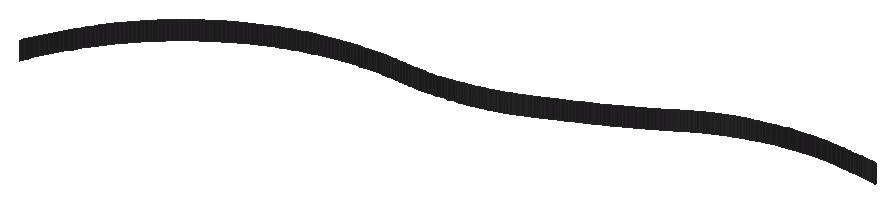
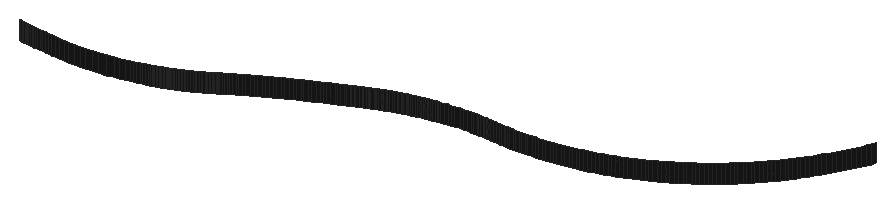
# SketchUp Ruby script. Lengths in inches.
U = 1.inch
M = Sketchup.active_model
def pt(a) = Geom::Point3d.new(a.map { |v| v * U })
def face(e, loops, mat)
  f = e.add_face(loops[0].map { |a| pt(a) })
  loops[1..].each { |l| e.add_face(l.map { |a| pt(a) }).erase! }
  f.material = f.back_material = mat if mat
  f
end
# faces: each face lists its corners as indices into pts; further lists are holes
def faces(e, pts, list, mat = nil) = list.each { |f| face(e, (f[0].is_a?(Array) ? f : [f]).map { |l| l.map { |i| pts[i] } }, mat) }
# xy, xz, yz: faces in a plane at the given z, y or x. An outline is a flat list of corners, or four numbers for a rectangle; further outlines are holes
def ring(l) = l.size == 4 ? [[l[0], l[1]], [l[2], l[1]], [l[2], l[3]], [l[0], l[3]]] : l.each_slice(2).to_a
def flat(e, list, mat, &to3) = list.each { |f| face(e, (f[0].is_a?(Array) ? f : [f]).map { |l| ring(l).map { |u, v| to3.(u, v) } }, mat) }
def xy(e, z, list, mat = nil) = flat(e, list, mat) { |x, y| [x, y, z] }
def xz(e, y, list, mat = nil) = flat(e, list, mat) { |x, z| [x, y, z] }
def yz(e, x, list, mat = nil) = flat(e, list, mat) { |y, z| [x, y, z] }
def lines(e, pts, list) = list.each { |a, b| e.add_line(pt(pts[a]), pt(pts[b])) }
# prism: a flat outline (further loops are holes) pulled along v
def prism(e, loops, v, mat = nil)
  f = face(e, loops, mat); d = Geom::Vector3d.new(v.map { |x| x * U })
  f.pushpull(f.normal.samedirection?(d) ? d.length : -d.length)
end
def box(e, o, s, mat = nil) = prism(e, [[o, [o[0] + s[0], o[1], o[2]], [o[0] + s[0], o[1] + s[1], o[2]], [o[0], o[1] + s[1], o[2]]]], [0, 0, s[2]], mat)
def at(x, y, z, deg = 0) = Geom::Transformation.translation(pt([x, y, z])) * Geom::Transformation.rotation(ORIGIN, Z_AXIS, deg.degrees)
def axes(o, x, y, z) = Geom::Transformation.new([*x, 0, *y, 0, *z, 0, *pt(o).to_a, 1])
def part(name) = M.definitions.add(name)
# library, detail: a bought-in or finely detailed component or shape, given as its bounding box
def library(name, o, s) = part(name).tap { |d| box(d.entities, o, s) }
def detail(e, o, s) = box(e.add_group.entities, o, s)
def put(e, d, t, mat = nil) = e.add_instance(d, t).tap { |i| i.material = mat if mat }
def group(e, t, mat = nil) = e.add_group.tap { |g| g.transformation = t; g.material = mat if mat }.entities
root = M.entities
M.materials.add("Marble_07_1K").color = [36, 34, 36]
xz(root,796.49,[[326.62,18,326.73,19],[326.73,18,326.84,19],[326.84,18,326.97,19]],"Marble_07_1K")
xz(root,796.5,[[326.25,18,326.34,19],[326.34,18,326.43,19],[326.43,18,326.52,19],[327.11,18,327.27,19]],"Marble_07_1K")
xz(root,796.51,[[326.07,18,326.16,19]],"Marble_07_1K")
xz(root,796.52,[[325.9,18,325.99,19]],"Marble_07_1K")
xz(root,796.53,[[325.73,18,325.82,19]],"Marble_07_1K")
xz(root,796.55,[[324.45,18,324.62,19],[325.4375,18,325.54,19]],"Marble_07_1K")
xz(root,796.56,[[324.78,18,324.93,19],[324.93,18,325.08,19],[325.08,18,325.21,19],[325.21,18,325.33,19]],"Marble_07_1K")
xz(root,802.3,[[347.43,18,347.47,19]],"Marble_07_1K")
xz(root,802.33,[[347.24,18,347.28,19]],"Marble_07_1K")
xz(root,802.34,[[347.16,18,347.2,19]],"Marble_07_1K")
xz(root,802.35,[[347.09,18,347.125,19]],"Marble_07_1K")
xz(root,802.36,[[347.01,18,347.05,19]],"Marble_07_1K")
xz(root,802.38,[[346.85,18,346.89,19]],"Marble_07_1K")
xz(root,802.39,[[346.74,18,346.8,19]],"Marble_07_1K")
xz(root,802.52,[[344.29,18,344.58,19]],"Marble_07_1K")
p = [[312.07,787.94,18],[311.99,787.75,18],[311.99,787.75,19],[312.07,787.94,19],[312.16,788.14,18],[312.16,788.14,19],
  [312.26,788.35,18],[312.26,788.35,19],[312.37,788.56,18],[312.37,788.56,19],[312.48,788.77,18],[312.48,788.77,19],
  [312.6,788.98,18],[312.6,788.98,19],[312.72,789.19,18],[312.72,789.19,19],[312.83,789.39,18],[312.83,789.39,19],
  [312.95,789.59,18],[312.95,789.59,19],[313.0625,789.78,18],[313.0625,789.78,19],[313.17,789.96,18],[313.17,789.96,19],
  [313.28,790.13,18],[313.28,790.13,19],[313.39,790.29,18],[313.39,790.29,19],[313.49,790.45,18],[313.49,790.45,19],
  [313.6,790.6,18],[313.6,790.6,19],[313.7,790.75,18],[313.7,790.75,19],[313.8125,790.9,18],[313.8125,790.9,19],
  [313.92,791.05,18],[313.92,791.05,19],[314.03,791.19,18],[314.03,791.19,19],[314.15,791.34,18],[314.15,791.34,19],
  [314.26,791.48,18],[314.26,791.48,19],[314.38,791.62,18],[314.38,791.62,19],[314.5,791.76,18],[314.5,791.76,19],
  [314.62,791.9,18],[314.62,791.9,19],[314.74,792.04,18],[314.74,792.04,19],[314.87,792.17,18],[314.87,792.17,19],
  [314.99,792.3,18],[314.99,792.3,19],[315.12,792.43,18],[315.12,792.43,19],[315.25,792.5625,18],[315.25,792.5625,19],
  [315.38,792.69,18],[315.38,792.69,19],[315.51,792.82,18],[315.51,792.82,19],[315.65,792.94,18],[315.65,792.94,19],
  [315.79,793.0625,18],[315.79,793.0625,19],[315.92,793.19,18],[315.92,793.19,19],[316.0625,793.3,18],[316.0625,793.3,19],
  [316.2,793.42,18],[316.2,793.42,19],[316.35,793.54,18],[316.35,793.54,19],[316.49,793.65,18],[316.49,793.65,19],
  [316.64,793.76,18],[316.64,793.76,19],[316.78,793.87,18],[316.78,793.87,19],[316.93,793.98,18],[316.93,793.98,19],
  [317.08,794.08,18],[317.08,794.08,19],[317.23,794.1875,18],[317.23,794.1875,19],[317.39,794.29,18],[317.39,794.29,19],
  [317.54,794.39,18],[317.54,794.39,19],[317.7,794.48,18],[317.7,794.48,19],[317.85,794.58,18],[317.85,794.58,19],
  [318.01,794.67,18],[318.01,794.67,19],[318.17,794.76,18],[318.17,794.76,19],[318.33,794.85,18],[318.33,794.85,19],
  [318.49,794.94,18],[318.49,794.94,19],[318.65,795.03,18],[318.65,795.03,19],[318.82,795.11,18],[318.82,795.11,19],
  [318.98,795.1875,18],[318.98,795.1875,19],[319.15,795.27,18],[319.15,795.27,19],[319.32,795.34,18],[319.32,795.34,19],
  [319.48,795.42,18],[319.48,795.42,19],[319.65,795.49,18],[319.65,795.49,19],[319.82,795.56,18],[319.82,795.56,19],
  [319.99,795.625,18],[319.99,795.625,19],[320.16,795.69,18],[320.16,795.69,19],[320.34,795.75,18],[320.34,795.75,19],
  [320.51,795.8125,18],[320.51,795.8125,19],[320.68,795.87,18],[320.68,795.87,19],[320.86,795.93,18],[320.86,795.93,19],
  [321.03,795.98,18],[321.03,795.98,19],[321.21,796.03,18],[321.21,796.03,19],[321.39,796.08,18],[321.39,796.08,19],
  [321.5625,796.125,18],[321.5625,796.125,19],[321.74,796.17,18],[321.74,796.17,19],[321.92,796.21,18],[321.92,796.21,19],
  [322.1,796.25,18],[322.1,796.25,19],[322.28,796.29,18],[322.28,796.29,19],[322.46,796.32,18],[322.46,796.32,19],
  [322.64,796.36,18],[322.64,796.36,19],[322.82,796.39,18],[322.82,796.39,19],[323,796.41,18],[323,796.41,19],
  [323.18,796.4375,18],[323.18,796.4375,19],[323.37,796.46,18],[323.37,796.46,19],[323.55,796.48,18],[323.55,796.48,19],
  [323.73,796.5,18],[323.73,796.5,19],[323.92,796.51,18],[323.92,796.51,19],[324.1,796.53,18],[324.1,796.53,19],
  [324.28,796.54,18],[324.28,796.54,19],[324.45,796.55,18],[324.45,796.55,19],[325.64,796.54,18],[325.54,796.55,18],
  [325.54,796.55,19],[325.64,796.54,19],[325.73,796.53,18],[325.73,796.53,19],[325.9,796.52,18],[325.82,796.53,18],
  [325.82,796.53,19],[325.9,796.52,19],[326.07,796.51,18],[325.99,796.52,18],[325.99,796.52,19],[326.07,796.51,19],
  [326.25,796.5,18],[326.16,796.51,18],[326.16,796.51,19],[326.25,796.5,19],[326.62,796.49,18],[326.52,796.5,18],
  [326.52,796.5,19],[326.62,796.49,19],[327.11,796.5,18],[326.97,796.49,18],[326.97,796.49,19],[327.11,796.5,19],
  [327.45,796.51,18],[327.27,796.5,18],[327.27,796.5,19],[327.45,796.51,19],[327.65,796.52,18],[327.65,796.52,19],
  [327.88,796.53,18],[327.88,796.53,19],[328.11,796.56,18],[328.11,796.56,19],[324.78,796.56,18],[324.62,796.55,18],
  [324.62,796.55,19],[324.78,796.56,19],[325.4375,796.55,18],[325.33,796.56,18],[325.33,796.56,19],[325.4375,796.55,19],
  [328.3125,796.58,18],[328.3125,796.58,19],[328.49,796.6,18],[328.49,796.6,19],[328.65,796.625,18],[328.65,796.625,19],
  [328.79,796.65,18],[328.79,796.65,19],[328.91,796.67,18],[328.91,796.67,19],[329.02,796.68,18],[329.02,796.68,19],
  [329.13,796.7,18],[329.13,796.7,19],[329.23,796.72,18],[329.23,796.72,19],[329.32,796.74,18],[329.32,796.74,19],
  [329.41,796.76,18],[329.41,796.76,19],[329.5,796.77,18],[329.5,796.77,19],[329.58,796.79,18],[329.58,796.79,19],
  [329.66,796.81,18],[329.66,796.81,19],[329.82,796.85,18],[329.74,796.83,18],[329.74,796.83,19],[329.82,796.85,19],
  [329.9,796.87,18],[329.9,796.87,19],[329.98,796.89,18],[329.98,796.89,19],[330.0625,796.91,18],[330.0625,796.91,19],
  [330.22,796.95,18],[330.14,796.93,18],[330.14,796.93,19],[330.22,796.95,19],[330.3,796.97,18],[330.3,796.97,19],
  [330.38,796.99,18],[330.38,796.99,19],[330.46,797.01,18],[330.46,797.01,19],[330.62,797.06,18],[330.54,797.04,18],
  [330.54,797.04,19],[330.62,797.06,19],[330.69,797.08,18],[330.69,797.08,19],[330.77,797.11,18],[330.77,797.11,19],
  [330.85,797.13,18],[330.85,797.13,19],[330.93,797.16,18],[330.93,797.16,19],[331.01,797.1875,18],[331.01,797.1875,19],
  [331.08,797.21,18],[331.08,797.21,19],[331.16,797.24,18],[331.16,797.24,19],[331.24,797.27,18],[331.24,797.27,19],
  [331.32,797.29,18],[331.32,797.29,19],[331.39,797.32,18],[331.39,797.32,19],[331.47,797.35,18],[331.47,797.35,19],
  [331.62,797.41,18],[331.55,797.38,18],[331.55,797.38,19],[331.62,797.41,19],[331.7,797.44,18],[331.7,797.44,19],
  [331.78,797.47,18],[331.78,797.47,19],[331.85,797.5,18],[331.85,797.5,19],[332,797.57,18],[331.93,797.54,18],
  [331.93,797.54,19],[332,797.57,19],[332.08,797.6,18],[332.08,797.6,19],[332.15,797.63,18],[332.15,797.63,19],
  [332.23,797.67,18],[332.23,797.67,19],[332.31,797.7,18],[332.31,797.7,19],[332.38,797.74,18],[332.38,797.74,19],
  [332.46,797.77,18],[332.46,797.77,19],[332.625,797.85,18],[332.54,797.8125,18],[332.54,797.8125,19],[332.625,797.85,19],
  [332.71,797.9,18],[332.71,797.9,19],[332.81,797.94,18],[332.81,797.94,19],[332.91,797.99,18],[332.91,797.99,19],
  [333.02,798.04,18],[333.02,798.04,19],[333.14,798.1,18],[333.14,798.1,19],[333.27,798.16,18],[333.27,798.16,19],
  [333.41,798.22,18],[333.41,798.22,19],[333.55,798.29,18],[333.55,798.29,19],[333.7,798.36,18],[333.7,798.36,19],
  [333.85,798.43,18],[333.85,798.43,19],[334.01,798.5,18],[334.01,798.5,19],[334.16,798.57,18],[334.16,798.57,19],
  [334.31,798.65,18],[334.31,798.65,19],[334.47,798.72,18],[334.47,798.72,19],[334.62,798.8,18],[334.62,798.8,19],
  [334.77,798.87,18],[334.77,798.87,19],[334.92,798.95,18],[334.92,798.95,19],[335.08,799.02,18],[335.08,799.02,19],
  [335.23,799.1,18],[335.23,799.1,19],[335.375,799.18,18],[335.375,799.18,19],[335.53,799.26,18],[335.53,799.26,19],
  [335.68,799.34,18],[335.68,799.34,19],[335.83,799.42,18],[335.83,799.42,19],[335.97,799.5,18],[335.97,799.5,19],
  [336.12,799.58,18],[336.12,799.58,19],[336.27,799.66,18],[336.27,799.66,19],[336.42,799.75,18],[336.42,799.75,19],
  [336.57,799.83,18],[336.57,799.83,19],[336.71,799.91,18],[336.71,799.91,19],[336.86,800,18],[336.86,800,19],
  [337,800.08,18],[337,800.08,19],[337.13,800.16,18],[337.13,800.16,19],[337.26,800.23,18],[337.26,800.23,19],
  [337.375,800.3,18],[337.375,800.3,19],[337.48,800.37,18],[337.48,800.37,19],[337.57,800.42,18],[337.57,800.42,19],
  [337.65,800.47,18],[337.65,800.47,19],[337.78,800.54,18],[337.72,800.51,18],[337.72,800.51,19],[337.78,800.54,19],
  [337.82,800.57,18],[337.82,800.57,19],[337.86,800.6,18],[337.86,800.6,19],[337.95,800.66,18],[337.93,800.64,18],
  [337.93,800.64,19],[337.95,800.66,19],[337.89,800.62,18],[337.89,800.62,19],[338.07,800.73,18],[338.04,800.71,18],
  [338.04,800.71,19],[338.07,800.73,19],[338.01,800.7,18],[338.01,800.7,19],[337.98,800.68,18],[337.98,800.68,19],
  [338.11,800.75,18],[338.11,800.75,19],[338.17,800.8,18],[338.14,800.77,18],[338.14,800.77,19],[338.17,800.8,19],
  [338.25,800.84,18],[338.21,800.82,18],[338.21,800.82,19],[338.25,800.84,19],[338.29,800.87,18],[338.29,800.87,19],
  [338.39,800.92,18],[338.34,800.89,18],[338.34,800.89,19],[338.39,800.92,19],[338.45,800.96,18],[338.45,800.96,19],
  [338.59,801.04,18],[338.52,801,18],[338.52,801,19],[338.59,801.04,19],[338.68,801.09,18],[338.68,801.09,19],
  [338.77,801.13,18],[338.77,801.13,19],[338.85,801.17,18],[338.85,801.17,19],[338.92,801.21,18],[338.92,801.21,19],
  [338.98,801.24,18],[338.98,801.24,19],[339.03,801.27,18],[339.03,801.27,19],[339.08,801.29,18],[339.08,801.29,19],
  [339.17,801.33,18],[339.125,801.3125,18],[339.125,801.3125,19],[339.17,801.33,19],[339.21,801.35,18],[339.21,801.35,19],
  [339.28,801.39,18],[339.24,801.37,18],[339.24,801.37,19],[339.28,801.39,19],[339.38,801.43,18],[339.35,801.42,18],
  [339.35,801.42,19],[339.38,801.43,19],[339.3125,801.4,18],[339.3125,801.4,19],[339.44,801.46,18],[339.41,801.45,18],
  [339.41,801.45,19],[339.44,801.46,19],[339.48,801.48,18],[339.48,801.48,19],[339.57,801.52,18],[339.54,801.5,18],
  [339.54,801.5,19],[339.57,801.52,19],[339.51,801.49,18],[339.51,801.49,19],[339.67,801.56,18],[339.64,801.54,18],
  [339.64,801.54,19],[339.67,801.56,19],[339.61,801.53,18],[339.61,801.53,19],[339.77,801.6,18],[339.74,801.59,18],
  [339.74,801.59,19],[339.77,801.6,19],[339.71,801.57,18],[339.71,801.57,19],[339.87,801.64,18],[339.84,801.625,18],
  [339.84,801.625,19],[339.87,801.64,19],[339.8,801.61,18],[339.8,801.61,19],[339.9,801.65,18],[339.9,801.65,19],
  [339.97,801.68,18],[339.94,801.66,18],[339.94,801.66,19],[339.97,801.68,19],[340.07,801.71,18],[340.03,801.7,18],
  [340.03,801.7,19],[340.07,801.71,19],[340,801.69,18],[340,801.69,19],[340.17,801.75,18],[340.13,801.74,18],
  [340.13,801.74,19],[340.17,801.75,19],[340.1,801.73,18],[340.1,801.73,19],[340.27,801.79,18],[340.23,801.77,18],
  [340.23,801.77,19],[340.27,801.79,19],[340.2,801.76,18],[340.2,801.76,19],[340.37,801.82,18],[340.33,801.81,18],
  [340.33,801.81,19],[340.37,801.82,19],[340.3,801.8,18],[340.3,801.8,19],[340.47,801.86,18],[340.44,801.84,18],
  [340.44,801.84,19],[340.47,801.86,19],[340.4,801.83,18],[340.4,801.83,19],[340.57,801.89,18],[340.54,801.88,18],
  [340.54,801.88,19],[340.57,801.89,19],[340.5,801.87,18],[340.5,801.87,19],[340.66,801.92,18],[340.61,801.9,18],
  [340.61,801.9,19],[340.66,801.92,19],[340.79,801.95,18],[340.72,801.93,18],[340.72,801.93,19],[340.79,801.95,19],
  [340.87,801.97,18],[340.87,801.97,19],[340.96,802,18],[340.96,802,19],[341.07,802.03,18],[341.07,802.03,19],
  [341.21,802.07,18],[341.21,802.07,19],[341.36,802.11,18],[341.36,802.11,19],[341.55,802.15,18],[341.55,802.15,19],
  [341.76,802.2,18],[341.76,802.2,19],[342.01,802.26,18],[342.01,802.26,19],[342.3,802.32,18],[342.3,802.32,19],
  [342.63,802.39,18],[342.63,802.39,19],[347.16,802.34,18],[347.125,802.35,18],[347.125,802.35,19],[347.16,802.34,19],
  [347.24,802.33,18],[347.2,802.34,18],[347.2,802.34,19],[347.24,802.33,19],[347.35,802.3125,18],[347.32,802.32,18],
  [347.32,802.32,19],[347.35,802.3125,19],[347.28,802.33,18],[347.28,802.33,19],[347.43,802.3,18],[347.39,802.31,18],
  [347.39,802.31,19],[347.43,802.3,19],[342.99,802.4375,18],[342.99,802.4375,19],[343.34,802.47,18],[343.34,802.47,19],
  [346.1,802.45,18],[345.9375,802.46,18],[345.9375,802.46,19],[346.1,802.45,19],[346.25,802.4375,18],[346.25,802.4375,19],
  [346.38,802.43,18],[346.38,802.43,19],[346.49,802.42,18],[346.49,802.42,19],[346.59,802.41,18],[346.59,802.41,19],
  [346.67,802.4,18],[346.67,802.4,19],[346.74,802.39,18],[346.74,802.39,19],[346.85,802.38,18],[346.8,802.39,18],
  [346.8,802.39,19],[346.85,802.38,19],[346.97,802.37,18],[346.93,802.375,18],[346.93,802.375,19],[346.97,802.37,19],
  [346.89,802.38,18],[346.89,802.38,19],[347.09,802.35,18],[347.05,802.36,18],[347.05,802.36,19],[347.09,802.35,19],
  [347.01,802.36,18],[347.01,802.36,19],[343.67,802.5,18],[343.67,802.5,19],[343.99,802.51,18],[343.99,802.51,19],
  [344.29,802.52,18],[344.29,802.52,19],[344.85,802.51,18],[344.58,802.52,18],[344.58,802.52,19],[344.85,802.51,19],
  [345.11,802.5,18],[345.11,802.5,19],[345.34,802.49,18],[345.34,802.49,19],[345.56,802.48,18],[345.56,802.48,19],
  [345.76,802.47,18],[345.76,802.47,19]]
faces(root,p,[[0,1,2,3],[4,0,3,5],[6,4,5,7],[8,6,7,9],[10,8,9,11],[12,10,11,13],[14,12,13,15],[16,14,15,17],
  [18,16,17,19],[20,18,19,21],[22,20,21,23],[24,22,23,25],[26,24,25,27],[28,26,27,29],[30,28,29,31],[32,30,31,33],
  [34,32,33,35],[36,34,35,37],[38,36,37,39],[40,38,39,41],[42,40,41,43],[44,42,43,45],[46,44,45,47],[48,46,47,49],
  [50,48,49,51],[52,50,51,53],[54,52,53,55],[56,54,55,57],[58,56,57,59],[60,58,59,61],[62,60,61,63],[64,62,63,65],
  [66,64,65,67],[68,66,67,69],[70,68,69,71],[72,70,71,73],[74,72,73,75],[76,74,75,77],[78,76,77,79],[80,78,79,81],
  [82,80,81,83],[84,82,83,85],[86,84,85,87],[88,86,87,89],[90,88,89,91],[92,90,91,93],[94,92,93,95],[96,94,95,97],
  [98,96,97,99],[100,98,99,101],[102,100,101,103],[104,102,103,105],[106,104,105,107],[108,106,107,109],[110,108,109,111],[112,110,111,113],
  [114,112,113,115],[116,114,115,117],[118,116,117,119],[120,118,119,121],[122,120,121,123],[124,122,123,125],[126,124,125,127],[128,126,127,129],
  [130,128,129,131],[132,130,131,133],[134,132,133,135],[136,134,135,137],[138,136,137,139],[140,138,139,141],[142,140,141,143],[144,142,143,145],
  [146,144,145,147],[148,146,147,149],[150,148,149,151],[152,150,151,153],[154,152,153,155],[156,154,155,157],[158,156,157,159],[160,158,159,161],
  [162,160,161,163],[164,162,163,165],[166,164,165,167],[168,166,167,169],[170,168,169,171],[172,173,174,175],[176,172,175,177],[178,179,180,181],
  [182,183,184,185],[186,187,188,189],[190,191,192,193],[194,195,196,197],[198,199,200,201],[202,198,201,203],[204,202,203,205],[206,204,205,207],
  [208,209,210,211],[212,213,214,215],[216,206,207,217],[218,216,217,219],[220,218,219,221],[222,220,221,223],[224,222,223,225],[226,224,225,227],
  [228,226,227,229],[230,228,229,231],[232,230,231,233],[234,232,233,235],[236,234,235,237],[238,236,237,239],[240,238,239,241],[242,243,244,245],
  [243,240,241,244],[246,242,245,247],[248,246,247,249],[250,248,249,251],[252,253,254,255],[253,250,251,254],[256,252,255,257],[258,256,257,259],
  [260,258,259,261],[262,263,264,265],[263,260,261,264],[266,262,265,267],[268,266,267,269],[270,268,269,271],[272,270,271,273],[274,272,273,275],
  [276,274,275,277],[278,276,277,279],[280,278,279,281],[282,280,281,283],[284,282,283,285],[286,284,285,287],[288,289,290,291],[289,286,287,290],
  [292,288,291,293],[294,292,293,295],[296,294,295,297],[298,299,300,301],[299,296,297,300],[302,298,301,303],[304,302,303,305],[306,304,305,307],
  [308,306,307,309],[310,308,309,311],[312,310,311,313],[314,315,316,317],[315,312,313,316],[318,314,317,319],[320,318,319,321],[322,320,321,323],
  [324,322,323,325],[326,324,325,327],[328,326,327,329],[330,328,329,331],[332,330,331,333],[334,332,333,335],[336,334,335,337],[338,336,337,339],
  [340,338,339,341],[342,340,341,343],[344,342,343,345],[346,344,345,347],[348,346,347,349],[350,348,349,351],[352,350,351,353],[354,352,353,355],
  [356,354,355,357],[358,356,357,359],[360,358,359,361],[362,360,361,363],[364,362,363,365],[366,364,365,367],[368,366,367,369],[370,368,369,371],
  [372,370,371,373],[374,372,373,375],[376,374,375,377],[378,376,377,379],[380,378,379,381],[382,380,381,383],[384,382,383,385],[386,384,385,387],
  [388,386,387,389],[390,388,389,391],[392,393,394,395],[393,390,391,394],[396,392,395,397],[398,396,397,399],[400,401,402,403],[401,404,405,402],
  [404,398,399,405],[406,407,408,409],[407,410,411,408],[410,412,413,411],[412,400,403,413],[414,406,409,415],[416,417,418,419],[417,414,415,418],
  [420,421,422,423],[421,416,419,422],[424,420,423,425],[426,427,428,429],[427,424,425,428],[430,426,429,431],[432,433,434,435],[433,430,431,434],
  [436,432,435,437],[438,436,437,439],[440,438,439,441],[442,440,441,443],[444,442,443,445],[446,444,445,447],[448,446,447,449],[450,451,452,453],
  [451,448,449,452],[454,450,453,455],[456,457,458,459],[457,454,455,458],[460,461,462,463],[461,464,465,462],[464,456,459,465],[466,467,468,469],
  [467,460,463,468],[470,466,469,471],[472,473,474,475],[473,476,477,474],[476,470,471,477],[478,479,480,481],[479,482,483,480],[482,472,475,483],
  [484,485,486,487],[485,488,489,486],[488,478,481,489],[490,491,492,493],[491,494,495,492],[494,484,487,495],[496,490,493,497],[498,499,500,501],
  [499,496,497,500],[502,503,504,505],[503,506,507,504],[506,498,501,507],[508,509,510,511],[509,512,513,510],[512,502,505,513],[514,515,516,517],
  [515,518,519,516],[518,508,511,519],[520,521,522,523],[521,524,525,522],[524,514,517,525],[526,527,528,529],[527,530,531,528],[530,520,523,531],
  [532,533,534,535],[533,536,537,534],[536,526,529,537],[538,539,540,541],[539,532,535,540],[542,543,544,545],[543,538,541,544],[546,542,545,547],
  [548,546,547,549],[550,548,549,551],[552,550,551,553],[554,552,553,555],[556,554,555,557],[558,556,557,559],[560,558,559,561],[562,560,561,563],
  [564,562,563,565],[566,567,568,569],[570,571,572,573],[574,575,576,577],[575,578,579,576],[580,581,582,583],[581,574,577,582],[584,564,565,585],
  [586,584,585,587],[588,589,590,591],[592,588,591,593],[594,592,593,595],[596,594,595,597],[598,596,597,599],[600,598,599,601],[602,600,601,603],
  [604,605,606,607],[608,609,610,611],[609,612,613,610],[614,615,616,617],[618,608,611,619],[620,586,587,621],[622,620,621,623],[624,622,623,625],
  [626,627,628,629],[630,626,629,631],[632,630,631,633],[634,632,633,635],[636,634,635,637],[589,636,637,590]],"Marble_07_1K")
